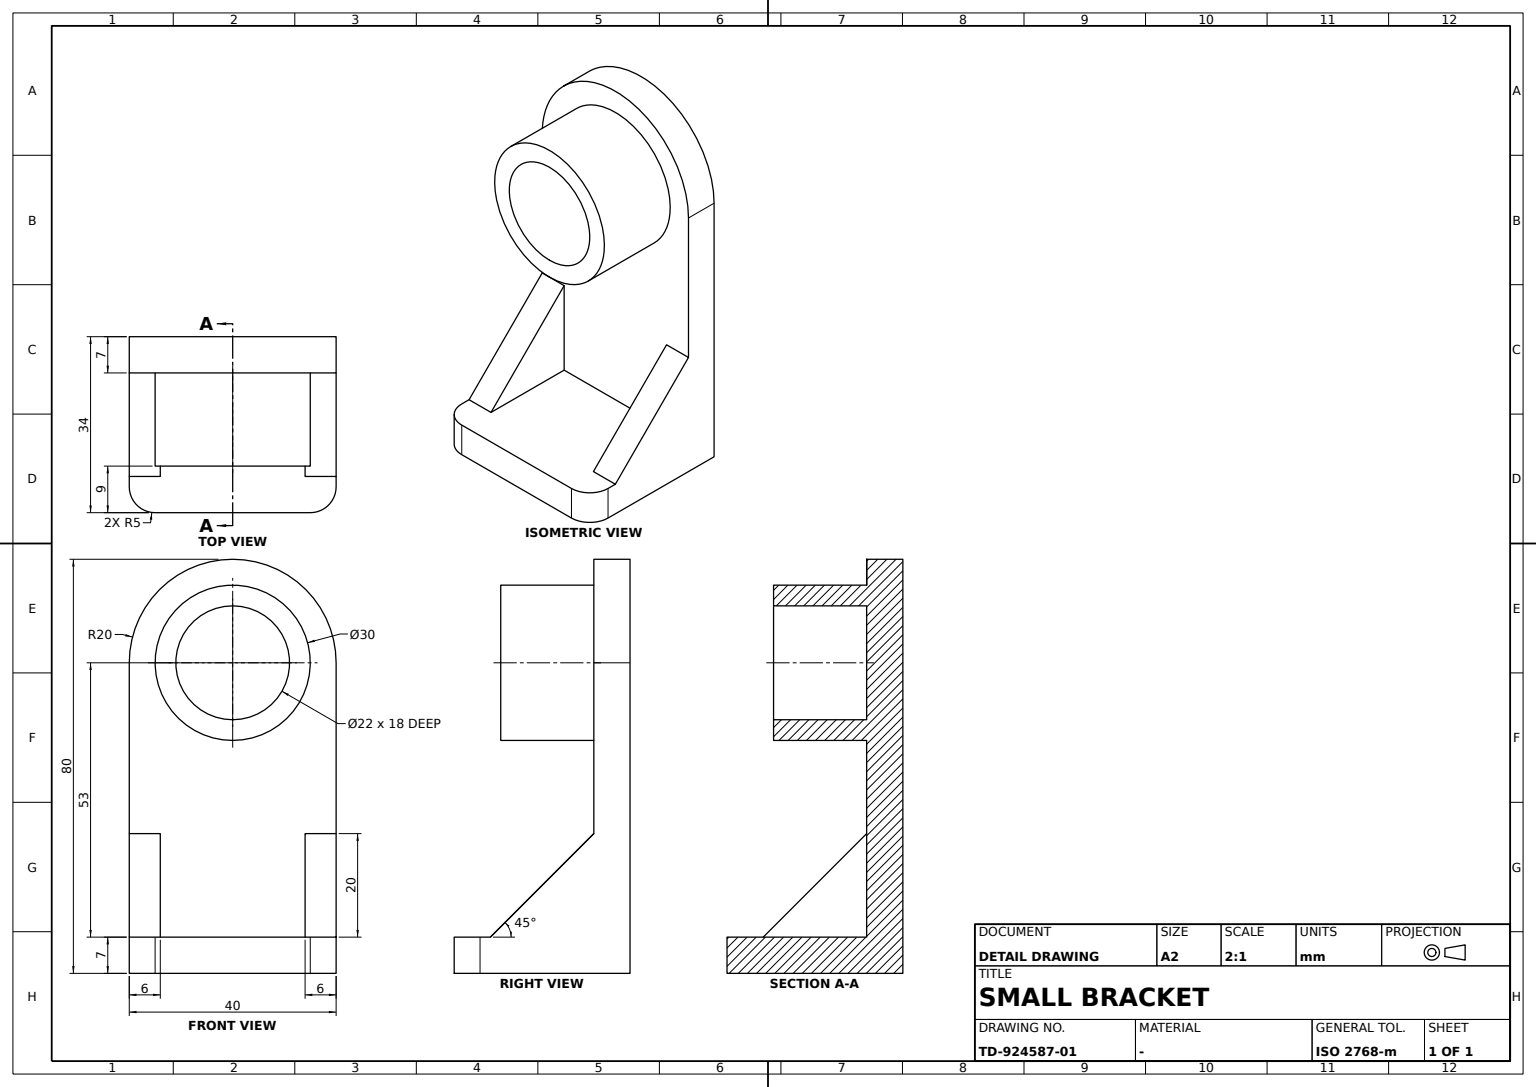
ISO-10303-21;
HEADER;
FILE_DESCRIPTION((''),'2;1');
FILE_NAME('','',(''),(''),'','','');
FILE_SCHEMA(('AUTOMOTIVE_DESIGN'));
ENDSEC;
DATA;
#1=APPLICATION_CONTEXT('');
#2=PRODUCT_CONTEXT('',#1,'mechanical');
#3=PRODUCT('','','',(#2));
#4=PRODUCT_DEFINITION_FORMATION('','',#3);
#5=PRODUCT_DEFINITION_CONTEXT('',#1,'design');
#6=PRODUCT_DEFINITION('','',#4,#5);
#7=PRODUCT_DEFINITION_SHAPE('','',#6);
#8=(LENGTH_UNIT()NAMED_UNIT(*)SI_UNIT(.MILLI.,.METRE.));
#9=(NAMED_UNIT(*)PLANE_ANGLE_UNIT()SI_UNIT($,.RADIAN.));
#10=(NAMED_UNIT(*)SI_UNIT($,.STERADIAN.)SOLID_ANGLE_UNIT());
#11=UNCERTAINTY_MEASURE_WITH_UNIT(LENGTH_MEASURE(0.005),#8,'distance_accuracy_value','');
#12=(GEOMETRIC_REPRESENTATION_CONTEXT(3)GLOBAL_UNCERTAINTY_ASSIGNED_CONTEXT((#11))GLOBAL_UNIT_ASSIGNED_CONTEXT((#8,#9,#10))REPRESENTATION_CONTEXT('',''));
#13=CARTESIAN_POINT('',(29.,-20.,0.));
#14=VERTEX_POINT('',#13);
#15=CARTESIAN_POINT('',(29.,-20.,7.));
#16=VERTEX_POINT('',#15);
#17=CARTESIAN_POINT('',(29.,-20.,3.5));
#18=DIRECTION('',(0.,0.,1.));
#19=VECTOR('',#18,1000.);
#20=LINE('',#17,#19);
#21=EDGE_CURVE('',#14,#16,#20,.T.);
#22=ORIENTED_EDGE('',*,*,#21,.F.);
#23=CARTESIAN_POINT('',(34.,-15.,0.));
#24=VERTEX_POINT('',#23);
#25=CARTESIAN_POINT('',(29.,-15.,0.));
#26=DIRECTION('',(1.,0.,0.));
#27=AXIS2_PLACEMENT_3D('',#25,#18,#26);
#28=CIRCLE('',#27,5.);
#29=EDGE_CURVE('',#14,#24,#28,.T.);
#30=ORIENTED_EDGE('',*,*,#29,.T.);
#31=CARTESIAN_POINT('',(34.,-15.,7.));
#32=VERTEX_POINT('',#31);
#33=CARTESIAN_POINT('',(34.,-15.,3.5));
#34=LINE('',#33,#19);
#35=EDGE_CURVE('',#24,#32,#34,.T.);
#36=ORIENTED_EDGE('',*,*,#35,.T.);
#37=CARTESIAN_POINT('',(29.,-15.,7.));
#38=AXIS2_PLACEMENT_3D('',#37,#18,#26);
#39=CIRCLE('',#38,5.);
#40=EDGE_CURVE('',#16,#32,#39,.T.);
#41=ORIENTED_EDGE('',*,*,#40,.F.);
#42=EDGE_LOOP('',(#22,#30,#36,#41));
#43=FACE_BOUND('',#42,.T.);
#44=CARTESIAN_POINT('',(29.,-15.,3.5));
#45=AXIS2_PLACEMENT_3D('',#44,#18,#26);
#46=CYLINDRICAL_SURFACE('',#45,5.);
#47=ADVANCED_FACE('',(#43),#46,.T.);
#48=CARTESIAN_POINT('',(0.,20.,0.));
#49=VERTEX_POINT('',#48);
#50=CARTESIAN_POINT('',(0.,20.,60.));
#51=VERTEX_POINT('',#50);
#52=LINE('',#48,#19);
#53=EDGE_CURVE('',#49,#51,#52,.T.);
#54=ORIENTED_EDGE('',*,*,#53,.F.);
#55=CARTESIAN_POINT('',(0.,-20.,0.));
#56=VERTEX_POINT('',#55);
#57=CARTESIAN_POINT('',(0.,0.,0.));
#58=DIRECTION('',(0.,1.,0.));
#59=VECTOR('',#58,1000.);
#60=LINE('',#57,#59);
#61=EDGE_CURVE('',#56,#49,#60,.T.);
#62=ORIENTED_EDGE('',*,*,#61,.F.);
#63=CARTESIAN_POINT('',(0.,-20.,60.));
#64=VERTEX_POINT('',#63);
#65=LINE('',#55,#19);
#66=EDGE_CURVE('',#56,#64,#65,.T.);
#67=ORIENTED_EDGE('',*,*,#66,.T.);
#68=CARTESIAN_POINT('',(0.,0.,60.));
#69=DIRECTION('',(0.,0.,-1.));
#70=AXIS2_PLACEMENT_3D('',#68,#26,#69);
#71=CIRCLE('',#70,20.);
#72=EDGE_CURVE('',#51,#64,#71,.T.);
#73=ORIENTED_EDGE('',*,*,#72,.F.);
#74=EDGE_LOOP('',(#54,#62,#67,#73));
#75=FACE_BOUND('',#74,.T.);
#76=AXIS2_PLACEMENT_3D('',#55,#26,#58);
#77=PLANE('',#76);
#78=ADVANCED_FACE('',(#75),#77,.F.);
#79=CARTESIAN_POINT('',(25.,0.,45.));
#80=VERTEX_POINT('',#79);
#81=CARTESIAN_POINT('',(25.,0.,60.));
#82=AXIS2_PLACEMENT_3D('',#81,#26,#69);
#83=CIRCLE('',#82,15.);
#84=EDGE_CURVE('',#80,#80,#83,.T.);
#85=ORIENTED_EDGE('',*,*,#84,.T.);
#86=EDGE_LOOP('',(#85));
#87=FACE_BOUND('',#86,.T.);
#88=CARTESIAN_POINT('',(25.,0.,49.));
#89=VERTEX_POINT('',#88);
#90=CIRCLE('',#82,11.);
#91=EDGE_CURVE('',#89,#89,#90,.T.);
#92=ORIENTED_EDGE('',*,*,#91,.F.);
#93=EDGE_LOOP('',(#92));
#94=FACE_BOUND('',#93,.T.);
#95=CARTESIAN_POINT('',(25.,0.,0.));
#96=AXIS2_PLACEMENT_3D('',#95,#26,#58);
#97=PLANE('',#96);
#98=ADVANCED_FACE('',(#87,#94),#97,.T.);
#99=CARTESIAN_POINT('',(27.,14.,7.));
#100=VERTEX_POINT('',#99);
#101=CARTESIAN_POINT('',(7.,14.,7.));
#102=VERTEX_POINT('',#101);
#103=CARTESIAN_POINT('',(0.,14.,7.));
#104=DIRECTION('',(-1.,0.,0.));
#105=VECTOR('',#104,1000.);
#106=LINE('',#103,#105);
#107=EDGE_CURVE('',#100,#102,#106,.T.);
#108=ORIENTED_EDGE('',*,*,#107,.F.);
#109=CARTESIAN_POINT('',(7.,14.,27.));
#110=VERTEX_POINT('',#109);
#111=DIRECTION('',(0.707106781,0.,-0.707106781));
#112=VECTOR('',#111,1000.);
#113=LINE('',#109,#112);
#114=EDGE_CURVE('',#110,#100,#113,.T.);
#115=ORIENTED_EDGE('',*,*,#114,.F.);
#116=CARTESIAN_POINT('',(7.,14.,0.));
#117=LINE('',#116,#19);
#118=EDGE_CURVE('',#102,#110,#117,.T.);
#119=ORIENTED_EDGE('',*,*,#118,.F.);
#120=EDGE_LOOP('',(#108,#115,#119));
#121=FACE_BOUND('',#120,.T.);
#122=CARTESIAN_POINT('',(0.,14.,0.));
#123=AXIS2_PLACEMENT_3D('',#122,#58,#104);
#124=PLANE('',#123);
#125=ADVANCED_FACE('',(#121),#124,.F.);
#126=CARTESIAN_POINT('',(34.,15.,0.));
#127=VERTEX_POINT('',#126);
#128=CARTESIAN_POINT('',(29.,20.,0.));
#129=VERTEX_POINT('',#128);
#130=CARTESIAN_POINT('',(29.,15.,0.));
#131=AXIS2_PLACEMENT_3D('',#130,#18,#26);
#132=CIRCLE('',#131,5.);
#133=EDGE_CURVE('',#127,#129,#132,.T.);
#134=ORIENTED_EDGE('',*,*,#133,.F.);
#135=CARTESIAN_POINT('',(34.,0.,0.));
#136=DIRECTION('',(0.,-1.,0.));
#137=VECTOR('',#136,1000.);
#138=LINE('',#135,#137);
#139=EDGE_CURVE('',#127,#24,#138,.T.);
#140=ORIENTED_EDGE('',*,*,#139,.T.);
#141=ORIENTED_EDGE('',*,*,#29,.F.);
#142=LINE('',#55,#105);
#143=EDGE_CURVE('',#14,#56,#142,.T.);
#144=ORIENTED_EDGE('',*,*,#143,.T.);
#145=ORIENTED_EDGE('',*,*,#61,.T.);
#146=VECTOR('',#26,1000.);
#147=LINE('',#48,#146);
#148=EDGE_CURVE('',#49,#129,#147,.T.);
#149=ORIENTED_EDGE('',*,*,#148,.T.);
#150=EDGE_LOOP('',(#134,#140,#141,#144,#145,#149));
#151=FACE_BOUND('',#150,.T.);
#152=AXIS2_PLACEMENT_3D('',#57,#18,#58);
#153=PLANE('',#152);
#154=ADVANCED_FACE('',(#151),#153,.F.);
#155=ORIENTED_EDGE('',*,*,#133,.T.);
#156=CARTESIAN_POINT('',(29.,20.,7.));
#157=VERTEX_POINT('',#156);
#158=CARTESIAN_POINT('',(29.,20.,3.5));
#159=LINE('',#158,#19);
#160=EDGE_CURVE('',#129,#157,#159,.T.);
#161=ORIENTED_EDGE('',*,*,#160,.T.);
#162=CARTESIAN_POINT('',(34.,15.,7.));
#163=VERTEX_POINT('',#162);
#164=CARTESIAN_POINT('',(29.,15.,7.));
#165=AXIS2_PLACEMENT_3D('',#164,#18,#26);
#166=CIRCLE('',#165,5.);
#167=EDGE_CURVE('',#163,#157,#166,.T.);
#168=ORIENTED_EDGE('',*,*,#167,.F.);
#169=CARTESIAN_POINT('',(34.,15.,3.5));
#170=LINE('',#169,#19);
#171=EDGE_CURVE('',#127,#163,#170,.T.);
#172=ORIENTED_EDGE('',*,*,#171,.F.);
#173=EDGE_LOOP('',(#155,#161,#168,#172));
#174=FACE_BOUND('',#173,.T.);
#175=CARTESIAN_POINT('',(29.,15.,3.5));
#176=AXIS2_PLACEMENT_3D('',#175,#18,#58);
#177=CYLINDRICAL_SURFACE('',#176,5.);
#178=ADVANCED_FACE('',(#174),#177,.T.);
#179=CARTESIAN_POINT('',(7.,20.,27.));
#180=VERTEX_POINT('',#179);
#181=CARTESIAN_POINT('',(27.,20.,7.));
#182=VERTEX_POINT('',#181);
#183=CARTESIAN_POINT('',(17.,20.,17.));
#184=LINE('',#183,#112);
#185=EDGE_CURVE('',#180,#182,#184,.T.);
#186=ORIENTED_EDGE('',*,*,#185,.F.);
#187=LINE('',#179,#137);
#188=EDGE_CURVE('',#180,#110,#187,.T.);
#189=ORIENTED_EDGE('',*,*,#188,.T.);
#190=ORIENTED_EDGE('',*,*,#114,.T.);
#191=CARTESIAN_POINT('',(27.,0.,7.));
#192=LINE('',#191,#137);
#193=EDGE_CURVE('',#182,#100,#192,.T.);
#194=ORIENTED_EDGE('',*,*,#193,.F.);
#195=EDGE_LOOP('',(#186,#189,#190,#194));
#196=FACE_BOUND('',#195,.T.);
#197=DIRECTION('',(-0.707106781,0.,-0.707106781));
#198=AXIS2_PLACEMENT_3D('',#179,#197,#111);
#199=PLANE('',#198);
#200=ADVANCED_FACE('',(#196),#199,.F.);
#201=ORIENTED_EDGE('',*,*,#167,.T.);
#202=CARTESIAN_POINT('',(0.,20.,7.));
#203=LINE('',#202,#146);
#204=EDGE_CURVE('',#182,#157,#203,.T.);
#205=ORIENTED_EDGE('',*,*,#204,.F.);
#206=ORIENTED_EDGE('',*,*,#193,.T.);
#207=ORIENTED_EDGE('',*,*,#107,.T.);
#208=CARTESIAN_POINT('',(7.,-14.,7.));
#209=VERTEX_POINT('',#208);
#210=CARTESIAN_POINT('',(7.,0.,7.));
#211=LINE('',#210,#59);
#212=EDGE_CURVE('',#209,#102,#211,.T.);
#213=ORIENTED_EDGE('',*,*,#212,.F.);
#214=CARTESIAN_POINT('',(27.,-14.,7.));
#215=VERTEX_POINT('',#214);
#216=CARTESIAN_POINT('',(0.,-14.,7.));
#217=LINE('',#216,#105);
#218=EDGE_CURVE('',#215,#209,#217,.T.);
#219=ORIENTED_EDGE('',*,*,#218,.F.);
#220=CARTESIAN_POINT('',(27.,-20.,7.));
#221=VERTEX_POINT('',#220);
#222=LINE('',#181,#59);
#223=EDGE_CURVE('',#221,#215,#222,.T.);
#224=ORIENTED_EDGE('',*,*,#223,.F.);
#225=CARTESIAN_POINT('',(0.,-20.,7.));
#226=LINE('',#225,#105);
#227=EDGE_CURVE('',#16,#221,#226,.T.);
#228=ORIENTED_EDGE('',*,*,#227,.F.);
#229=ORIENTED_EDGE('',*,*,#40,.T.);
#230=CARTESIAN_POINT('',(34.,0.,7.));
#231=LINE('',#230,#137);
#232=EDGE_CURVE('',#163,#32,#231,.T.);
#233=ORIENTED_EDGE('',*,*,#232,.F.);
#234=EDGE_LOOP('',(#201,#205,#206,#207,#213,#219,#224,#228,#229,#233));
#235=FACE_BOUND('',#234,.T.);
#236=CARTESIAN_POINT('',(0.,0.,7.));
#237=AXIS2_PLACEMENT_3D('',#236,#18,#58);
#238=PLANE('',#237);
#239=ADVANCED_FACE('',(#235),#238,.T.);
#240=CARTESIAN_POINT('',(7.,20.,60.));
#241=VERTEX_POINT('',#240);
#242=CARTESIAN_POINT('',(7.,-20.,60.));
#243=VERTEX_POINT('',#242);
#244=CARTESIAN_POINT('',(7.,0.,60.));
#245=AXIS2_PLACEMENT_3D('',#244,#26,#69);
#246=CIRCLE('',#245,20.);
#247=EDGE_CURVE('',#241,#243,#246,.T.);
#248=ORIENTED_EDGE('',*,*,#247,.F.);
#249=CARTESIAN_POINT('',(3.5,20.,60.));
#250=LINE('',#249,#146);
#251=EDGE_CURVE('',#51,#241,#250,.T.);
#252=ORIENTED_EDGE('',*,*,#251,.F.);
#253=ORIENTED_EDGE('',*,*,#72,.T.);
#254=CARTESIAN_POINT('',(3.5,-20.,60.));
#255=LINE('',#254,#146);
#256=EDGE_CURVE('',#64,#243,#255,.T.);
#257=ORIENTED_EDGE('',*,*,#256,.T.);
#258=EDGE_LOOP('',(#248,#252,#253,#257));
#259=FACE_BOUND('',#258,.T.);
#260=CARTESIAN_POINT('',(3.5,0.,60.));
#261=AXIS2_PLACEMENT_3D('',#260,#26,#58);
#262=CYLINDRICAL_SURFACE('',#261,20.);
#263=ADVANCED_FACE('',(#259),#262,.T.);
#264=ORIENTED_EDGE('',*,*,#91,.T.);
#265=EDGE_LOOP('',(#264));
#266=FACE_BOUND('',#265,.T.);
#267=CARTESIAN_POINT('',(7.,0.,49.));
#268=VERTEX_POINT('',#267);
#269=CIRCLE('',#245,11.);
#270=EDGE_CURVE('',#268,#268,#269,.T.);
#271=ORIENTED_EDGE('',*,*,#270,.F.);
#272=EDGE_LOOP('',(#271));
#273=FACE_BOUND('',#272,.T.);
#274=CARTESIAN_POINT('',(16.,0.,60.));
#275=AXIS2_PLACEMENT_3D('',#274,#26,#58);
#276=CYLINDRICAL_SURFACE('',#275,11.);
#277=ADVANCED_FACE('',(#266,#273),#276,.F.);
#278=CARTESIAN_POINT('',(7.,-14.,27.));
#279=VERTEX_POINT('',#278);
#280=CARTESIAN_POINT('',(7.,-14.,0.));
#281=LINE('',#280,#19);
#282=EDGE_CURVE('',#209,#279,#281,.T.);
#283=ORIENTED_EDGE('',*,*,#282,.T.);
#284=LINE('',#278,#112);
#285=EDGE_CURVE('',#279,#215,#284,.T.);
#286=ORIENTED_EDGE('',*,*,#285,.T.);
#287=ORIENTED_EDGE('',*,*,#218,.T.);
#288=EDGE_LOOP('',(#283,#286,#287));
#289=FACE_BOUND('',#288,.T.);
#290=CARTESIAN_POINT('',(0.,-14.,0.));
#291=AXIS2_PLACEMENT_3D('',#290,#58,#104);
#292=PLANE('',#291);
#293=ADVANCED_FACE('',(#289),#292,.T.);
#294=CARTESIAN_POINT('',(7.,0.,45.));
#295=VERTEX_POINT('',#294);
#296=CIRCLE('',#245,15.);
#297=EDGE_CURVE('',#295,#295,#296,.T.);
#298=ORIENTED_EDGE('',*,*,#297,.T.);
#299=EDGE_LOOP('',(#298));
#300=FACE_BOUND('',#299,.T.);
#301=ORIENTED_EDGE('',*,*,#84,.F.);
#302=EDGE_LOOP('',(#301));
#303=FACE_BOUND('',#302,.T.);
#304=CYLINDRICAL_SURFACE('',#275,15.);
#305=ADVANCED_FACE('',(#300,#303),#304,.T.);
#306=ORIENTED_EDGE('',*,*,#66,.F.);
#307=ORIENTED_EDGE('',*,*,#143,.F.);
#308=ORIENTED_EDGE('',*,*,#21,.T.);
#309=ORIENTED_EDGE('',*,*,#227,.T.);
#310=CARTESIAN_POINT('',(7.,-20.,27.));
#311=VERTEX_POINT('',#310);
#312=LINE('',#310,#112);
#313=EDGE_CURVE('',#311,#221,#312,.T.);
#314=ORIENTED_EDGE('',*,*,#313,.F.);
#315=CARTESIAN_POINT('',(7.,-20.,0.));
#316=VECTOR('',#69,1000.);
#317=LINE('',#315,#316);
#318=EDGE_CURVE('',#243,#311,#317,.T.);
#319=ORIENTED_EDGE('',*,*,#318,.F.);
#320=ORIENTED_EDGE('',*,*,#256,.F.);
#321=EDGE_LOOP('',(#306,#307,#308,#309,#314,#319,#320));
#322=FACE_BOUND('',#321,.T.);
#323=CARTESIAN_POINT('',(34.,-20.,0.));
#324=AXIS2_PLACEMENT_3D('',#323,#58,#104);
#325=PLANE('',#324);
#326=ADVANCED_FACE('',(#322),#325,.F.);
#327=ORIENTED_EDGE('',*,*,#270,.T.);
#328=EDGE_LOOP('',(#327));
#329=FACE_BOUND('',#328,.T.);
#330=CARTESIAN_POINT('',(7.,0.,0.));
#331=AXIS2_PLACEMENT_3D('',#330,#26,#58);
#332=PLANE('',#331);
#333=ADVANCED_FACE('',(#329),#332,.T.);
#334=ORIENTED_EDGE('',*,*,#285,.F.);
#335=CARTESIAN_POINT('',(7.,0.,27.));
#336=LINE('',#335,#59);
#337=EDGE_CURVE('',#311,#279,#336,.T.);
#338=ORIENTED_EDGE('',*,*,#337,.F.);
#339=ORIENTED_EDGE('',*,*,#313,.T.);
#340=ORIENTED_EDGE('',*,*,#223,.T.);
#341=EDGE_LOOP('',(#334,#338,#339,#340));
#342=FACE_BOUND('',#341,.T.);
#343=ADVANCED_FACE('',(#342),#199,.F.);
#344=ORIENTED_EDGE('',*,*,#232,.T.);
#345=ORIENTED_EDGE('',*,*,#35,.F.);
#346=ORIENTED_EDGE('',*,*,#139,.F.);
#347=ORIENTED_EDGE('',*,*,#171,.T.);
#348=EDGE_LOOP('',(#344,#345,#346,#347));
#349=FACE_BOUND('',#348,.T.);
#350=CARTESIAN_POINT('',(34.,20.,0.));
#351=AXIS2_PLACEMENT_3D('',#350,#104,#136);
#352=PLANE('',#351);
#353=ADVANCED_FACE('',(#349),#352,.F.);
#354=CARTESIAN_POINT('',(7.,20.,0.));
#355=LINE('',#354,#19);
#356=EDGE_CURVE('',#180,#241,#355,.T.);
#357=ORIENTED_EDGE('',*,*,#356,.F.);
#358=ORIENTED_EDGE('',*,*,#185,.T.);
#359=ORIENTED_EDGE('',*,*,#204,.T.);
#360=ORIENTED_EDGE('',*,*,#160,.F.);
#361=ORIENTED_EDGE('',*,*,#148,.F.);
#362=ORIENTED_EDGE('',*,*,#53,.T.);
#363=ORIENTED_EDGE('',*,*,#251,.T.);
#364=EDGE_LOOP('',(#357,#358,#359,#360,#361,#362,#363));
#365=FACE_BOUND('',#364,.T.);
#366=AXIS2_PLACEMENT_3D('',#48,#136,#26);
#367=PLANE('',#366);
#368=ADVANCED_FACE('',(#365),#367,.F.);
#369=ORIENTED_EDGE('',*,*,#297,.F.);
#370=EDGE_LOOP('',(#369));
#371=FACE_BOUND('',#370,.T.);
#372=ORIENTED_EDGE('',*,*,#212,.T.);
#373=ORIENTED_EDGE('',*,*,#118,.T.);
#374=ORIENTED_EDGE('',*,*,#188,.F.);
#375=ORIENTED_EDGE('',*,*,#356,.T.);
#376=ORIENTED_EDGE('',*,*,#247,.T.);
#377=ORIENTED_EDGE('',*,*,#318,.T.);
#378=ORIENTED_EDGE('',*,*,#337,.T.);
#379=ORIENTED_EDGE('',*,*,#282,.F.);
#380=EDGE_LOOP('',(#372,#373,#374,#375,#376,#377,#378,#379));
#381=FACE_BOUND('',#380,.T.);
#382=ADVANCED_FACE('',(#371,#381),#332,.T.);
#383=CLOSED_SHELL('',(#47,#78,#98,#125,#154,#178,#200,#239,#263,#277,#293,#305,#326,#333,#343,#353,#368,#382));
#384=MANIFOLD_SOLID_BREP('',#383);
#385=ADVANCED_BREP_SHAPE_REPRESENTATION('',(#384),#12);
#386=SHAPE_DEFINITION_REPRESENTATION(#7,#385);
ENDSEC;
END-ISO-10303-21;
